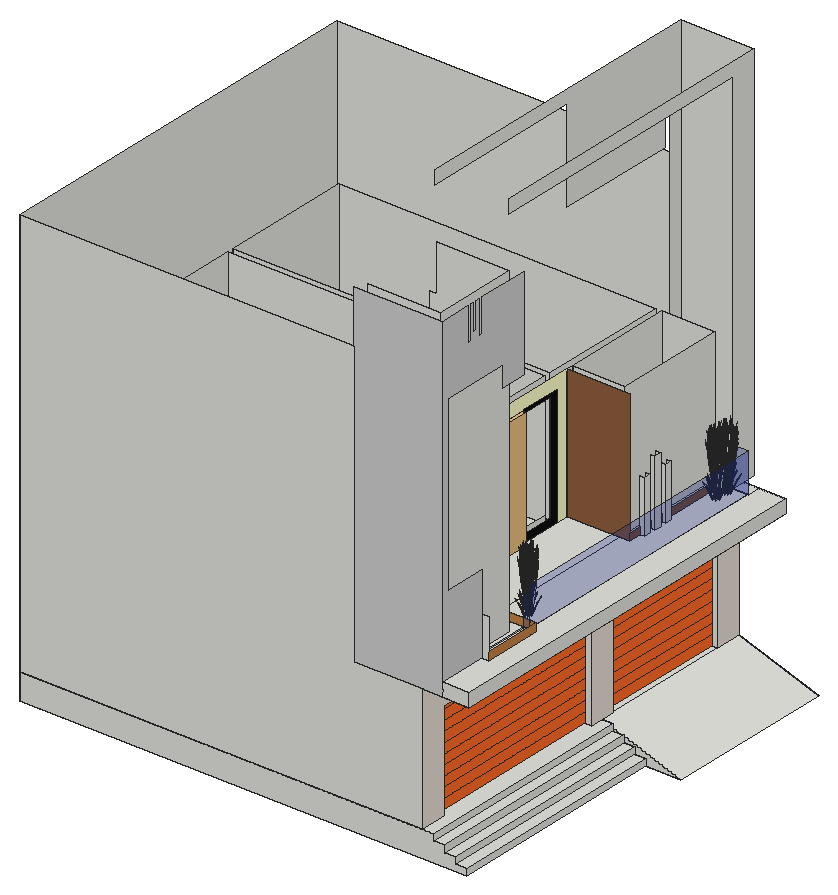
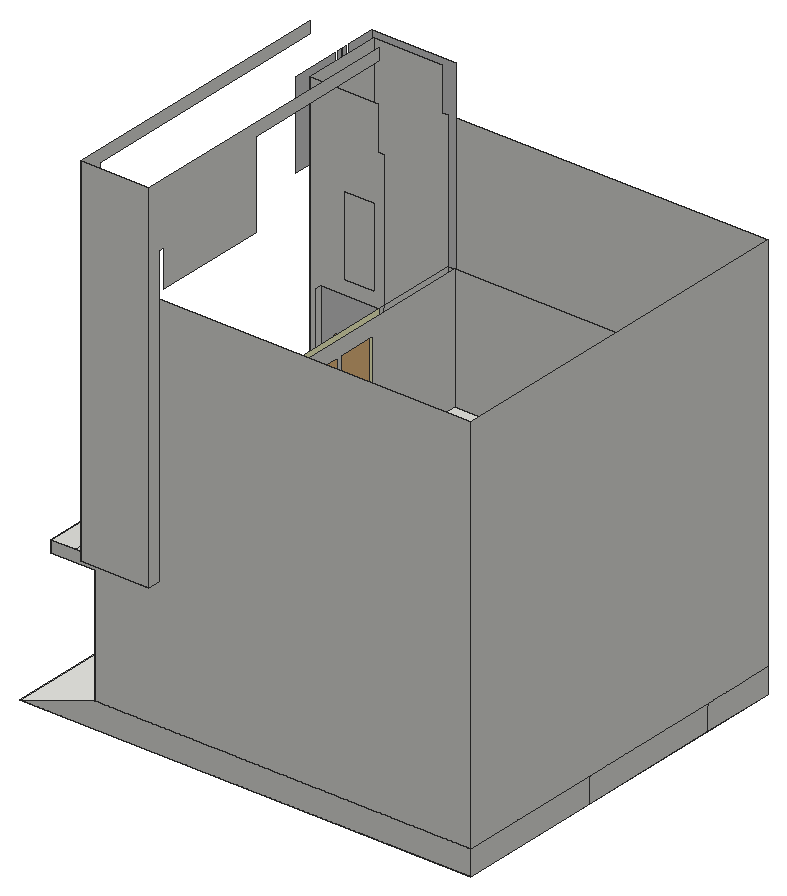
# SketchUp Ruby script. Lengths in inches.
U = 1.inch
M = Sketchup.active_model
def pt(a) = Geom::Point3d.new(a.map { |v| v * U })
def face(e, loops, mat)
  f = e.add_face(loops[0].map { |a| pt(a) })
  loops[1..].each { |l| e.add_face(l.map { |a| pt(a) }).erase! }
  f.material = f.back_material = mat if mat
  f
end
# faces: each face lists its corners as indices into pts; further lists are holes
def faces(e, pts, list, mat = nil) = list.each { |f| face(e, (f[0].is_a?(Array) ? f : [f]).map { |l| l.map { |i| pts[i] } }, mat) }
# xy, xz, yz: faces in a plane at the given z, y or x. An outline is a flat list of corners, or four numbers for a rectangle; further outlines are holes
def ring(l) = l.size == 4 ? [[l[0], l[1]], [l[2], l[1]], [l[2], l[3]], [l[0], l[3]]] : l.each_slice(2).to_a
def flat(e, list, mat, &to3) = list.each { |f| face(e, (f[0].is_a?(Array) ? f : [f]).map { |l| ring(l).map { |u, v| to3.(u, v) } }, mat) }
def xy(e, z, list, mat = nil) = flat(e, list, mat) { |x, y| [x, y, z] }
def xz(e, y, list, mat = nil) = flat(e, list, mat) { |x, z| [x, y, z] }
def yz(e, x, list, mat = nil) = flat(e, list, mat) { |y, z| [x, y, z] }
def lines(e, pts, list) = list.each { |a, b| e.add_line(pt(pts[a]), pt(pts[b])) }
# prism: a flat outline (further loops are holes) pulled along v
def prism(e, loops, v, mat = nil)
  f = face(e, loops, mat); d = Geom::Vector3d.new(v.map { |x| x * U })
  f.pushpull(f.normal.samedirection?(d) ? d.length : -d.length)
end
def box(e, o, s, mat = nil) = prism(e, [[o, [o[0] + s[0], o[1], o[2]], [o[0] + s[0], o[1] + s[1], o[2]], [o[0], o[1] + s[1], o[2]]]], [0, 0, s[2]], mat)
def at(x, y, z, deg = 0) = Geom::Transformation.translation(pt([x, y, z])) * Geom::Transformation.rotation(ORIGIN, Z_AXIS, deg.degrees)
def axes(o, x, y, z) = Geom::Transformation.new([*x, 0, *y, 0, *z, 0, *pt(o).to_a, 1])
def part(name) = M.definitions.add(name)
# library, detail: a bought-in or finely detailed component or shape, given as its bounding box
def library(name, o, s) = part(name).tap { |d| box(d.entities, o, s) }
def detail(e, o, s) = box(e.add_group.entities, o, s)
def put(e, d, t, mat = nil) = e.add_instance(d, t).tap { |i| i.material = mat if mat }
def group(e, t, mat = nil) = e.add_group.tap { |g| g.transformation = t; g.material = mat if mat }.entities
root = M.entities
M.materials.add("C05_Golden_Blaze").color = [255, 107, 39]
M.materials.add("E01_Mint_Frost").color = [255, 255, 204]
M.materials.add("Glass_Basic_01").color = [23, 48, 186]
M.materials["Glass_Basic_01"].alpha = 0.25
M.materials.add("LightPink_Translucent").color = [144, 107, 117]
M.materials["LightPink_Translucent"].alpha = 0.75
M.materials.add("Marble_01_1K").color = [230, 221, 211]
M.materials.add("ThomThom - ShoesRubber1").color = [15, 15, 15]
M.materials.add("Wood_Floor_01_1K").color = [196, 130, 70]
M.materials.add("Wood_Veneer_15_1K").color = [142, 95, 62]
M.materials.add("[Cladding_Siding_White]1").color = [207, 207, 207]
c1 = library("mesh-166",[-1553.69,-2604.3125,-42.18],[1702.88,1401.6,88.28])
c2 = part("Group17\#1")
put(c2.entities,c1,at(294.66,859.51,3.5))
c3 = library("porta+4",[0.2,-5.42,1.33],[46.55,4.72,83.21])
c4 = part("blade")
p = [[2.15,0.21,22],[0,0.17,0],[0.09,0.45,0],[2.18,0.31,22],[2.29,0.31,22],[0.38,0.45,0],
  [2.48,0.24,33],[2.49,0.24,33],[2.48,0.22,33]]
faces(c4.entities,p,[[0,1,2,3],[4,5,2,3],[6,3,4,7],[8,0,3,6]])
c5 = part("seeds")
p = [[0.3,-0.1,1.38],[-0.01,-0.03,1.59],[-0.01,-0.03,0.03],[0.14,-0.07,-0.07],[0.29,-0.03,3],[0.15,0.01,3.11]]
faces(c5.entities,p,[[0,1,2,3],[1,0,4,5]],"LightPink_Translucent")
c6 = part("blade with seeds")
put(c6.entities,c4,at(0,0,0))
put(c6.entities,c5,axes([2.4,0.25,30.99],[1.5799,-0.05474,1.17369],[-0.12525,1.92788,0.29478],[-0.07173,-0.02425,1.56792]))
xy(root,24,[[0,0,0,360,366,360,366,336,360,336,360,216,366,216,366,192,360,192,360,24,366,24,366,0]])
xy(root,114,[[360,24,366,192],[360,216,366,336]])
xy(root,138,[[366,0,408,360]])
xy(root,150,[[384,0,408,0,408,360,384,360,384,99,390,99,390,45,384,45],[9,9,297,225],[303,9,375,87],[303,93,351,243],[351,93,360,93,360,99,384,99,384,348,360,348,360,285,364,285,364,279,360,279,360,273,364,273,364,267,360,267,360,261,364,261,364,255,360,255,360,243,351,243],
  [9,231,297,351],[303,249,351,351],[370,348,384,360],[303,360,370,372]])
xz(root,0,[[0,24,366,24,366,138,303,138,303,396,0,396],[384,138,408,150]])
xz(root,0,[[303,138,384,444]],"[Cladding_Siding_White]1")
xz(root,9,[[9,150,297,270],[297,150,303,270],[303,150,303,402,309,402,309,444,375,444,375,150]])
xz(root,24,[[360,24,366,114]])
xz(root,45,[[384,150,390,186]])
xz(root,87,[[[303,150,375,150,375,444,309,444,309,402,303,402],[312,279,342,357],[312,153,342,231]]])
xz(root,93,[[303,150,303,270,360,270,360,150,345,150,345,234,309,234,309,150],[[309,150,345,234],[312,153,342,231]]],"[Cladding_Siding_White]1")
xz(root,99,[[360,150,384,157],[384,150,390,157]],"Wood_Floor_01_1K")
xz(root,192,[[360,24,366,114]])
xz(root,216,[[360,24,366,114]])
xz(root,225,[[9,150,297,270]])
xz(root,231,[[9,150,297,270]])
xz(root,243,[[303,150,360,270]],"Wood_Veneer_15_1K")
xz(root,249,[[303,150,351,270]])
xz(root,255,[[360,150,364,198]])
xz(root,261,[[360,150,364,198]])
xz(root,267,[[360,150,364,210]])
xz(root,273,[[360,150,364,210]])
xz(root,279,[[360,150,364,198]])
xz(root,285,[[360,150,364,198]])
xz(root,336,[[360,24,366,114]])
xz(root,348,[[360,150,370,186]])
xz(root,348,[[370,150,384,186]],"Glass_Basic_01")
xz(root,351,[[9,150,297,270],[303,150,351,270]])
xz(root,360,[[0,24,0,396,303,396,303,150,408,150,408,138,366,138,366,24]])
xz(root,372,[[303,150,370,498]])
yz(root,0,[[0,24,360,396]])
yz(root,9,[[9,150,225,270],[231,150,351,270]])
yz(root,297,[[[9,150,9,270,225,270,225,255.54,192,255.54,192,156.54,225,156.54,225,150],[108,156.54,147,255.54],[151,156.54,188,255.54]],[231,150,351,270]])
yz(root,303,[[9,150,87,270],[87,150,93,270],[360,150,360,438,354,438,354,402,243,402,243,486,93,486,93,498,372,498,372,150],[243,150,249,270],[249,150,351,270]])
yz(root,303,[[93,150,192,150,192,186.54,188,186.54,188,156.54,151,156.54,151,186.54,147,186.54,147,156.54,108,156.54,108,186.54,105,186.54,105,258.54,231,258.54,231,150,243,150,243,270,93,270]],"E01_Mint_Frost")
yz(root,303,[[192,150,231,150,231,258.51,192,258.51,192,255.54,225,255.54,225,156.54,192,156.54]],"ThomThom - ShoesRubber1")
yz(root,351,[[249,150,351,270]])
yz(root,360,[[93,150,99,270]])
yz(root,360,[[24,24,192,33],[216,24,336,33],[24,33,192,42],[216,33,336,42],[24,42,192,51],
  [216,42,336,51],[24,51,192,60],[216,51,336,60],[24,60,192,69],[216,60,336,69],
  [24,69,192,78],[216,69,336,78],[24,78,192,87],[216,78,336,87],[24,87,192,96],
  [216,87,336,96],[24,96,192,105],[216,96,336,105],[24,105,192,114],[216,105,336,114]],"C05_Golden_Blaze")
yz(root,360,[[243,150,255,156],[261,150,267,156],[273,150,279,156],[285,150,348,156]],"Wood_Veneer_15_1K")
yz(root,364,[[255,150,261,198],[267,150,273,210],[279,150,285,198]])
yz(root,366,[[0,24,24,24,24,114,192,114,192,24,216,24,216,114,336,114,336,24,360,24,360,138,0,138]],"Marble_01_1K")
yz(root,370,[[348,150,372,150,372,498,93,498,93,486,348,486]])
yz(root,375,[[9,150,87,444]])
yz(root,384,[[93,150,99,180],[99,150,348,186]],"Glass_Basic_01")
yz(root,384,[[0,150,45,150,45,222,6,222,6,378,69,378,69,360,93,360,93,444,45.12,444,45.12,414,41.79,414,41.79,444,38.45,444,38.45,420,35.12,420,35.12,444,31.79,444,31.79,414,28.45,414,28.45,444,0,444]],"[Cladding_Siding_White]1")
yz(root,390,[[45,150,99,157]],"Wood_Floor_01_1K")
yz(root,408,[[0,138,360,150]])
p = [[384,93,150],[390,93,150],[303,231,150],[303.15,190.71,150],[303.15,190.71,258.51],[360,242.96,150],
  [360,243,150],[360,255,150],[360,261,150],[360,267,150],[360,273,150],[360,279,150],
  [360,285,150]]
lines(root,p,[[0,1],[2,3],[3,4],[5,6],[7,8],[9,10],[11,12]])
g1 = group(root,at(0,0,0))
xy(g1,0,[[0,0,0,360,366,360,366,204,406,204,406,0],[366,204,438,360]])
xy(g1,6,[[396,0,406,204]])
xy(g1,12,[[386,0,396,204]])
xy(g1,18,[[376,0,386,204]])
xy(g1,24,[[0,0,376,0,376,204,366,204,366,360,0,360]])
xz(g1,0,[[0,0,406,0,406,6,396,6,396,12,386,12,386,18,376,18,376,24,0,24]])
xz(g1,204,[[366,0,406,6],[406,0,438,0,386,17.33,386,12,396,12,396,6,406,6],[366,6,396,12],[366,12,366,18,384,18,386,17.33,386,12],[386,17.33,384,18,386,18],
  [366,18,366,24,376,20.67,376,18],[376,18,376,20.67,384,18],[376,20.67,366,24,376,24]])
xz(g1,360,[[0,0,0,24,366,24,438,0]])
yz(g1,0,[[0,0,72,24],[72,0,216,24],[216,0,360,24]])
yz(g1,376,[[0,18,204,24]])
yz(g1,386,[[0,12,204,18]])
yz(g1,396,[[0,6,204,12]])
yz(g1,406,[[0,0,204,6]])
p = [[376,204,20.67],[384,204,18],[386,204,17.33],[438,204,0],[438,360,0],[366,360,24],
  [366,204,24]]
faces(g1,p,[[0,1,2,3,4,5,6]])
put(root,c2,axes([304.95,127.5625,285.12],[0,-0.05083,0],[0,0,0.07744],[-0.03937,0,0]))
put(root,c3,axes([310,97.01,148.65],[0.74,0,0],[0,0.74,0],[0,0,1.01007]))
put(root,c6,axes([370.13,327.31,151.97],[-0.2011,-0.61905,-0.65645],[0.5793,-0.22295,-0.17229],[-0.02223,-0.20963,1.449]))
put(root,c6,axes([371.39,112.01,151.97],[-0.2011,-0.61905,-0.65645],[0.5793,-0.22295,-0.17229],[-0.02223,-0.20963,1.449]))
put(root,c6,axes([371.39,338.93,151.97],[-0.2011,-0.61905,-0.65645],[0.5793,-0.22295,-0.17229],[-0.02223,-0.20963,1.449]))
put(root,c6,axes([371.97,328.36,151.97],[0.17956,0.55272,-0.65059],[-0.51723,0.19906,-0.17075],[0.01985,0.18717,1.43607]))
put(root,c6,axes([373.23,113.07,151.97],[0.17956,0.55272,-0.65059],[-0.51723,0.19906,-0.17075],[0.01985,0.18717,1.43607]))
put(root,c6,axes([373.23,339.99,151.97],[0.17956,0.55272,-0.65059],[-0.51723,0.19906,-0.17075],[0.01985,0.18717,1.43607]))
put(root,c6,axes([371.92,327.2,151.9375],[0.50939,0.09897,-0.58612],[-0.10749,0.61051,-0.15383],[0.15202,0.07398,1.29375]))
put(root,c6,axes([370.21,328.46,151.9375],[-0.50939,-0.09897,-0.58612],[0.10749,-0.61051,-0.15383],[-0.15202,-0.07398,1.29375]))
put(root,c6,axes([371.01,326.67,151.9375],[0.32983,-0.45375,-0.58612],[0.40974,0.41145,-0.15383],[0.13217,-0.11319,1.29375]))
put(root,c6,axes([371.12,328.99,151.9375],[-0.32983,0.45375,-0.58612],[-0.40974,-0.41145,-0.15383],[-0.13217,0.11319,1.29375]))
put(root,c6,axes([373.18,111.91,151.9375],[0.50939,0.09897,-0.58612],[-0.10749,0.61051,-0.15383],[0.15202,0.07398,1.29375]))
put(root,c6,axes([371.47,113.17,151.9375],[-0.50939,-0.09897,-0.58612],[0.10749,-0.61051,-0.15383],[-0.15202,-0.07398,1.29375]))
put(root,c6,axes([372.27,111.38,151.9375],[0.32983,-0.45375,-0.58612],[0.40974,0.41145,-0.15383],[0.13217,-0.11319,1.29375]))
put(root,c6,axes([372.375,113.7,151.9375],[-0.32983,0.45375,-0.58612],[-0.40974,-0.41145,-0.15383],[-0.13217,0.11319,1.29375]))
put(root,c6,axes([373.18,338.83,151.9375],[0.50939,0.09897,-0.58612],[-0.10749,0.61051,-0.15383],[0.15202,0.07398,1.29375]))
put(root,c6,axes([371.47,340.09,151.9375],[-0.50939,-0.09897,-0.58612],[0.10749,-0.61051,-0.15383],[-0.15202,-0.07398,1.29375]))
put(root,c6,axes([372.27,338.3,151.9375],[0.32983,-0.45375,-0.58612],[0.40974,0.41145,-0.15383],[0.13217,-0.11319,1.29375]))
put(root,c6,axes([372.375,340.62,151.9375],[-0.32983,0.45375,-0.58612],[-0.40974,-0.41145,-0.15383],[-0.13217,0.11319,1.29375]))
put(root,c6,axes([372.59,326.04,151.9],[0.4583,0.30184,-0.46672],[-0.27394,0.54125,0],[0.10438,0.06875,1.48054]))
put(root,c6,axes([371.66,330.23,151.9],[-0.4583,0.30184,-0.46672],[-0.27394,-0.54125,0],[-0.10438,0.06875,1.48054]))
put(root,c6,axes([368.95,327.22,151.9],[0,-0.60368,-0.46672],[0.54787,0,0],[0,-0.13749,1.48054]))
put(root,c6,axes([369.54,329.62,151.9],[-0.4583,-0.30184,-0.46672],[0.27394,-0.54125,0],[-0.10438,-0.06875,1.48054]))
put(root,c6,axes([370.47,325.43,151.9],[0.4583,-0.30184,-0.46672],[0.27394,0.54125,0],[0.10438,-0.06875,1.48054]))
put(root,c6,axes([373.18,328.4375,151.9],[0,0.60368,-0.46672],[-0.54787,0,0],[0,0.13749,1.48054]))
put(root,c6,axes([373.85,110.75,151.9],[0.4583,0.30184,-0.46672],[-0.27394,0.54125,0],[0.10438,0.06875,1.48054]))
put(root,c6,axes([372.92,114.94,151.9],[-0.4583,0.30184,-0.46672],[-0.27394,-0.54125,0],[-0.10438,0.06875,1.48054]))
put(root,c6,axes([370.21,111.93,151.9],[0,-0.60368,-0.46672],[0.54787,0,0],[0,-0.13749,1.48054]))
put(root,c6,axes([370.8,114.32,151.9],[-0.4583,-0.30184,-0.46672],[0.27394,-0.54125,0],[-0.10438,-0.06875,1.48054]))
put(root,c6,axes([371.73,110.14,151.9],[0.4583,-0.30184,-0.46672],[0.27394,0.54125,0],[0.10438,-0.06875,1.48054]))
put(root,c6,axes([374.44,113.15,151.9],[0,0.60368,-0.46672],[-0.54787,0,0],[0,0.13749,1.48054]))
put(root,c6,axes([373.85,337.67,151.9],[0.4583,0.30184,-0.46672],[-0.27394,0.54125,0],[0.10438,0.06875,1.48054]))
put(root,c6,axes([372.92,341.85,151.9],[-0.4583,0.30184,-0.46672],[-0.27394,-0.54125,0],[-0.10438,0.06875,1.48054]))
put(root,c6,axes([370.21,338.85,151.9],[0,-0.60368,-0.46672],[0.54787,0,0],[0,-0.13749,1.48054]))
put(root,c6,axes([370.8,341.24,151.9],[-0.4583,-0.30184,-0.46672],[0.27394,-0.54125,0],[-0.10438,-0.06875,1.48054]))
put(root,c6,axes([371.73,337.06,151.9],[0.4583,-0.30184,-0.46672],[0.27394,0.54125,0],[0.10438,-0.06875,1.48054]))
put(root,c6,axes([374.44,340.07,151.9],[0,0.60368,-0.46672],[-0.54787,0,0],[0,0.13749,1.48054]))
put(root,c6,axes([370.4375,327.47,152.08],[0.23759,-0.54397,-0.42055],[0.49367,0.26179,0.2024],[0,-0.12539,1.35025]))
put(root,c6,axes([370.47,328.27,152.08],[-0.29417,-0.5067,-0.42055],[0.44558,-0.35681,0.2024],[-0.0952,-0.0627,1.35025]))
put(root,c6,axes([371.65,327.39,152.08],[0.29417,0.5067,-0.42055],[-0.44558,0.35681,0.2024],[0.0952,0.0627,1.35025]))
put(root,c6,axes([371.69,328.19,152.08],[-0.23759,0.54397,-0.42055],[-0.49367,-0.26179,0.2024],[0,0.12539,1.35025]))
put(root,c6,axes([371.1,328.63,152.08],[-0.53176,0.03727,-0.42055],[-0.04809,-0.6186,0.2024],[-0.0952,0.0627,1.35025]))
put(root,c6,axes([371.7,112.17,152.08],[0.23759,-0.54397,-0.42055],[0.49367,0.26179,0.2024],[0,-0.12539,1.35025]))
put(root,c6,axes([371.73,112.98,152.08],[-0.29417,-0.5067,-0.42055],[0.44558,-0.35681,0.2024],[-0.0952,-0.0627,1.35025]))
put(root,c6,axes([372.91,112.1,152.08],[0.29417,0.5067,-0.42055],[-0.44558,0.35681,0.2024],[0.0952,0.0627,1.35025]))
put(root,c6,axes([372.95,112.9,152.08],[-0.23759,0.54397,-0.42055],[-0.49367,-0.26179,0.2024],[0,0.12539,1.35025]))
put(root,c6,axes([372.36,113.34,152.08],[-0.53176,0.03727,-0.42055],[-0.04809,-0.6186,0.2024],[-0.0952,0.0627,1.35025]))
put(root,c6,axes([371.7,339.09,152.08],[0.23759,-0.54397,-0.42055],[0.49367,0.26179,0.2024],[0,-0.12539,1.35025]))
put(root,c6,axes([371.73,339.89,152.08],[-0.29417,-0.5067,-0.42055],[0.44558,-0.35681,0.2024],[-0.0952,-0.0627,1.35025]))
put(root,c6,axes([372.91,339.02,152.08],[0.29417,0.5067,-0.42055],[-0.44558,0.35681,0.2024],[0.0952,0.0627,1.35025]))
put(root,c6,axes([372.95,339.82,152.08],[-0.23759,0.54397,-0.42055],[-0.49367,-0.26179,0.2024],[0,0.12539,1.35025]))
put(root,c6,axes([372.36,340.26,152.08],[-0.53176,0.03727,-0.42055],[-0.04809,-0.6186,0.2024],[-0.0952,0.0627,1.35025]))
put(root,c6,axes([370.58,325.67,151.91],[0.45686,0.14937,-0.29119],[-0.11503,0.52602,0.29119],[0.0921,-0.06066,1.30635]))
put(root,c6,axes([372.95,328.43,151.91],[-0.34183,0.37665,-0.29119],[-0.34183,-0.37665,0.29119],[0,0.12132,1.30635]))
put(root,c6,axes([369.67,329.39,151.91],[-0.11503,-0.52602,-0.29119],[0.45686,-0.14937,0.29119],[-0.0921,-0.06066,1.30635]))
put(root,c6,axes([371.55,329.99,151.91],[-0.45686,-0.14937,-0.29119],[0.11503,-0.52602,0.29119],[-0.0921,0.06066,1.30635]))
put(root,c6,axes([372.46,326.27,151.91],[0.11503,0.52602,-0.29119],[-0.45686,0.14937,0.29119],[0.0921,0.06066,1.30635]))
put(root,c6,axes([369.18,327.23,151.91],[0.34183,-0.37665,-0.29119],[0.34183,0.37665,0.29119],[0,-0.12132,1.30635]))
put(root,c6,axes([371.84,110.38,151.91],[0.45686,0.14937,-0.29119],[-0.11503,0.52602,0.29119],[0.0921,-0.06066,1.30635]))
put(root,c6,axes([374.21,113.13,151.91],[-0.34183,0.37665,-0.29119],[-0.34183,-0.37665,0.29119],[0,0.12132,1.30635]))
put(root,c6,axes([370.93,114.1,151.91],[-0.11503,-0.52602,-0.29119],[0.45686,-0.14937,0.29119],[-0.0921,-0.06066,1.30635]))
put(root,c6,axes([372.8125,114.7,151.91],[-0.45686,-0.14937,-0.29119],[0.11503,-0.52602,0.29119],[-0.0921,0.06066,1.30635]))
put(root,c6,axes([373.72,110.98,151.91],[0.11503,0.52602,-0.29119],[-0.45686,0.14937,0.29119],[0.0921,0.06066,1.30635]))
put(root,c6,axes([370.44,111.94,151.91],[0.34183,-0.37665,-0.29119],[0.34183,0.37665,0.29119],[0,-0.12132,1.30635]))
put(root,c6,axes([371.84,337.3,151.91],[0.45686,0.14937,-0.29119],[-0.11503,0.52602,0.29119],[0.0921,-0.06066,1.30635]))
put(root,c6,axes([374.21,340.05,151.91],[-0.34183,0.37665,-0.29119],[-0.34183,-0.37665,0.29119],[0,0.12132,1.30635]))
put(root,c6,axes([370.93,341.02,151.91],[-0.11503,-0.52602,-0.29119],[0.45686,-0.14937,0.29119],[-0.0921,-0.06066,1.30635]))
put(root,c6,axes([372.8125,341.62,151.91],[-0.45686,-0.14937,-0.29119],[0.11503,-0.52602,0.29119],[-0.0921,0.06066,1.30635]))
put(root,c6,axes([373.72,337.9,151.91],[0.11503,0.52602,-0.29119],[-0.45686,0.14937,0.29119],[0.0921,0.06066,1.30635]))
put(root,c6,axes([370.44,338.86,151.91],[0.34183,-0.37665,-0.29119],[0.34183,0.37665,0.29119],[0,-0.12132,1.30635]))
put(root,c6,axes([372.5625,330.34,151.4],[0.03568,-0.08715,1.65762],[0.44916,-0.25668,-0.25323],[0.13617,0.13285,0.28235]))
put(root,c6,axes([368.57,327.6,151.4],[0.01242,0.09514,1.65762],[-0.25036,0.49684,-0.25323],[-0.17783,-0.02504,0.28235]))
put(root,c6,axes([370.81,324.37,151.4],[-0.08214,0.02175,1.65762],[-0.45422,-0.24483,-0.25323],[0.00762,-0.20421,0.28235]))
put(root,c6,axes([370.47,330.32,151.4],[0.07925,-0.03285,1.65762],[0.47671,0.18081,-0.25323],[0.01394,0.20378,0.28235]))
put(root,c6,axes([373.86,327.69,151.4],[-0.02559,-0.09165,1.65762],[0.1775,-0.53611,-0.25323],[0.17905,-0.00771,0.28235]))
put(root,c6,axes([369.34,325.12,151.4],[-0.04743,0.07953,1.65762],[-0.47936,0.17146,-0.25323],[-0.1158,-0.15598,0.28235]))
put(root,c6,axes([368.4375,330.26,151.4],[0.06569,0.06031,1.65762],[0.11138,0.55882,-0.25323],[-0.14558,0.11917,0.28235]))
put(root,c6,axes([372.82,325.41,151.4],[-0.07329,-0.04756,1.65762],[-0.18827,-0.53132,-0.25323],[0.127,-0.14418,0.28235]))
put(root,c6,axes([373.82,115.05,151.4],[0.03568,-0.08715,1.65762],[0.44916,-0.25668,-0.25323],[0.13617,0.13285,0.28235]))
put(root,c6,axes([369.83,112.31,151.4],[0.01242,0.09514,1.65762],[-0.25036,0.49684,-0.25323],[-0.17783,-0.02504,0.28235]))
put(root,c6,axes([372.07,109.08,151.4],[-0.08214,0.02175,1.65762],[-0.45422,-0.24483,-0.25323],[0.00762,-0.20421,0.28235]))
put(root,c6,axes([371.73,115.03,151.4],[0.07925,-0.03285,1.65762],[0.47671,0.18081,-0.25323],[0.01394,0.20378,0.28235]))
put(root,c6,axes([375.12,112.4,151.4],[-0.02559,-0.09165,1.65762],[0.1775,-0.53611,-0.25323],[0.17905,-0.00771,0.28235]))
put(root,c6,axes([370.6,109.83,151.4],[-0.04743,0.07953,1.65762],[-0.47936,0.17146,-0.25323],[-0.1158,-0.15598,0.28235]))
put(root,c6,axes([369.7,114.97,151.4],[0.06569,0.06031,1.65762],[0.11138,0.55882,-0.25323],[-0.14558,0.11917,0.28235]))
put(root,c6,axes([374.08,110.12,151.4],[-0.07329,-0.04756,1.65762],[-0.18827,-0.53132,-0.25323],[0.127,-0.14418,0.28235]))
put(root,c6,axes([373.82,341.96,151.4],[0.03568,-0.08715,1.65762],[0.44916,-0.25668,-0.25323],[0.13617,0.13285,0.28235]))
put(root,c6,axes([369.83,339.23,151.4],[0.01242,0.09514,1.65762],[-0.25036,0.49684,-0.25323],[-0.17783,-0.02504,0.28235]))
put(root,c6,axes([372.07,336,151.4],[-0.08214,0.02175,1.65762],[-0.45422,-0.24483,-0.25323],[0.00762,-0.20421,0.28235]))
put(root,c6,axes([371.73,341.95,151.4],[0.07925,-0.03285,1.65762],[0.47671,0.18081,-0.25323],[0.01394,0.20378,0.28235]))
put(root,c6,axes([375.12,339.32,151.4],[-0.02559,-0.09165,1.65762],[0.1775,-0.53611,-0.25323],[0.17905,-0.00771,0.28235]))
put(root,c6,axes([370.6,336.75,151.4],[-0.04743,0.07953,1.65762],[-0.47936,0.17146,-0.25323],[-0.1158,-0.15598,0.28235]))
put(root,c6,axes([369.7,341.89,151.4],[0.06569,0.06031,1.65762],[0.11138,0.55882,-0.25323],[-0.14558,0.11917,0.28235]))
put(root,c6,axes([374.08,337.04,151.4],[-0.07329,-0.04756,1.65762],[-0.18827,-0.53132,-0.25323],[0.127,-0.14418,0.28235]))
put(root,c6,axes([370.09,326.75,151.5],[-0.482,0.24169,1.21193],[-0.15342,-0.69348,0.47091],[0.29598,0.01154,1.37843]))
put(root,c6,axes([371.35,111.46,151.5],[-0.482,0.24169,1.21193],[-0.15342,-0.69348,0.47091],[0.29598,0.01154,1.37843]))
put(root,c6,axes([371.35,338.38,151.5],[-0.482,0.24169,1.21193],[-0.15342,-0.69348,0.47091],[0.29598,0.01154,1.37843]))
put(root,c6,axes([371.47,328.46,152.51],[0.05706,0.68884,-0.2735],[-0.59432,0.04165,-0.47002],[-0.10465,0.09176,1.50125]))
put(root,c6,axes([371.75,327.74,152.51],[0.55148,0.28805,-0.2735],[-0.26554,0.60796,-0.47002],[0.01733,0.14927,1.50125]))
put(root,c6,axes([370.38,327.92,152.51],[-0.55148,-0.28805,-0.2735],[0.26554,-0.60796,-0.47002],[-0.01733,-0.14927,1.50125]))
put(root,c6,axes([370.65,327.2,152.51],[-0.05706,-0.68884,-0.2735],[0.59432,-0.04165,-0.47002],[0.10465,-0.09176,1.50125]))
put(root,c6,axes([371.34,327.11,152.51],[0.49442,-0.40079,-0.2735],[0.32878,0.56631,-0.47002],[0.12199,0.05751,1.50125]))
put(root,c6,axes([370.79,328.55,152.51],[-0.49442,0.40079,-0.2735],[-0.32878,-0.56631,-0.47002],[-0.12199,-0.05751,1.50125]))
put(root,c6,axes([372.73,113.17,152.51],[0.05706,0.68884,-0.2735],[-0.59432,0.04165,-0.47002],[-0.10465,0.09176,1.50125]))
put(root,c6,axes([373.01,112.45,152.51],[0.55148,0.28805,-0.2735],[-0.26554,0.60796,-0.47002],[0.01733,0.14927,1.50125]))
put(root,c6,axes([371.64,112.625,152.51],[-0.55148,-0.28805,-0.2735],[0.26554,-0.60796,-0.47002],[-0.01733,-0.14927,1.50125]))
put(root,c6,axes([371.91,111.9,152.51],[-0.05706,-0.68884,-0.2735],[0.59432,-0.04165,-0.47002],[0.10465,-0.09176,1.50125]))
put(root,c6,axes([372.6,111.82,152.51],[0.49442,-0.40079,-0.2735],[0.32878,0.56631,-0.47002],[0.12199,0.05751,1.50125]))
put(root,c6,axes([372.05,113.26,152.51],[-0.49442,0.40079,-0.2735],[-0.32878,-0.56631,-0.47002],[-0.12199,-0.05751,1.50125]))
put(root,c6,axes([372.73,340.09,152.51],[0.05706,0.68884,-0.2735],[-0.59432,0.04165,-0.47002],[-0.10465,0.09176,1.50125]))
put(root,c6,axes([373.01,339.37,152.51],[0.55148,0.28805,-0.2735],[-0.26554,0.60796,-0.47002],[0.01733,0.14927,1.50125]))
put(root,c6,axes([371.64,339.55,152.51],[-0.55148,-0.28805,-0.2735],[0.26554,-0.60796,-0.47002],[-0.01733,-0.14927,1.50125]))
put(root,c6,axes([371.91,338.82,152.51],[-0.05706,-0.68884,-0.2735],[0.59432,-0.04165,-0.47002],[0.10465,-0.09176,1.50125]))
put(root,c6,axes([372.6,338.74,152.51],[0.49442,-0.40079,-0.2735],[0.32878,0.56631,-0.47002],[0.12199,0.05751,1.50125]))
put(root,c6,axes([372.05,340.18,152.51],[-0.49442,0.40079,-0.2735],[-0.32878,-0.56631,-0.47002],[-0.12199,-0.05751,1.50125]))
put(root,c6,axes([371.64,329.15,152.05],[0.51411,-0.20483,-0.18046],[0.18065,0.59003,0.00007],[0.05675,-0.02264,1.63463]))
put(root,c6,axes([372.9,113.85,152.05],[0.51411,-0.20483,-0.18046],[0.18065,0.59003,0.00007],[0.05675,-0.02264,1.63463]))
put(root,c6,axes([372.9,340.77,152.05],[0.51411,-0.20483,-0.18046],[0.18065,0.59003,0.00007],[0.05675,-0.02264,1.63463]))
put(root,c6,axes([371.34,328.73,152.32],[-0.47817,-0.48589,-0.23681],[0.40236,-0.54561,0.51822],[-0.12876,0.05684,1.58123]))
put(root,c6,axes([372.6,113.44,152.32],[-0.47817,-0.48589,-0.23681],[0.40236,-0.54561,0.51822],[-0.12876,0.05684,1.58123]))
put(root,c6,axes([372.6,340.36,152.32],[-0.47817,-0.48589,-0.23681],[0.40236,-0.54561,0.51822],[-0.12876,0.05684,1.58123]))
put(root,c6,axes([370.52,328.56,152.29],[0.12979,-0.71533,-0.22023],[0.6154,0.12469,0.48194],[-0.10753,-0.09879,1.47054]))
put(root,c6,axes([371.78,113.27,152.29],[0.12979,-0.71533,-0.22023],[0.6154,0.12469,0.48194],[-0.10753,-0.09879,1.47054]))
put(root,c6,axes([371.78,340.19,152.29],[0.12979,-0.71533,-0.22023],[0.6154,0.12469,0.48194],[-0.10753,-0.09879,1.47054]))
put(root,c6,axes([370.72,324.8,152],[-0.3384,0.34633,-0.03659],[-0.31006,-0.3793,-0.1659],[-0.02183,-0.10747,0.54722]))
put(root,c6,axes([369.04,325.43,152],[-0.14126,0.49294,-0.03659],[-0.43477,-0.15163,-0.1659],[-0.06601,-0.08063,0.54722]))
put(root,c6,axes([371.99,109.51,152],[-0.3384,0.34633,-0.03659],[-0.31006,-0.3793,-0.1659],[-0.02183,-0.10747,0.54722]))
put(root,c6,axes([370.3,110.14,152],[-0.14126,0.49294,-0.03659],[-0.43477,-0.15163,-0.1659],[-0.06601,-0.08063,0.54722]))
put(root,c6,axes([371.99,336.42,152],[-0.3384,0.34633,-0.03659],[-0.31006,-0.3793,-0.1659],[-0.02183,-0.10747,0.54722]))
put(root,c6,axes([370.3,337.05,152],[-0.14126,0.49294,-0.03659],[-0.43477,-0.15163,-0.1659],[-0.06601,-0.08063,0.54722]))
put(root,c6,axes([374.09,327.56,152.125],[-0.3036,-0.38602,-0.06098],[0.3325,-0.3537,-0.27651],[0.09421,-0.0249,0.91203]))
put(root,c6,axes([375.35,112.27,152.125],[-0.3036,-0.38602,-0.06098],[0.3325,-0.3537,-0.27651],[0.09421,-0.0249,0.91203]))
put(root,c6,axes([375.35,339.1875,152.125],[-0.3036,-0.38602,-0.06098],[0.3325,-0.3537,-0.27651],[0.09421,-0.0249,0.91203]))
put(root,c6,axes([373.51,328.07,151.86],[-0.3154,0.07245,1.33088],[-0.0502,-0.57666,0.07618],[0.2209,-0.08728,0.75732]))
put(root,c6,axes([374.77,112.78,151.86],[-0.3154,0.07245,1.33088],[-0.0502,-0.57666,0.07618],[0.2209,-0.08728,0.75732]))
put(root,c6,axes([374.77,339.7,151.86],[-0.3154,0.07245,1.33088],[-0.0502,-0.57666,0.07618],[0.2209,-0.08728,0.75732]))
put(root,c6,axes([371.69,330.06,152.0625],[-0.30235,-0.60704,-0.04834],[0.51222,-0.33735,0.48511],[-0.12622,0.0578,1.53813]))
put(root,c6,axes([372.95,114.77,152.0625],[-0.30235,-0.60704,-0.04834],[0.51222,-0.33735,0.48511],[-0.12622,0.0578,1.53813]))
put(root,c6,axes([372.95,341.69,152.0625],[-0.30235,-0.60704,-0.04834],[0.51222,-0.33735,0.48511],[-0.12622,0.0578,1.53813]))
put(root,c6,axes([373.07,328.33,152.07],[-0.61202,-0.00483,-0.04678],[0,-0.67471,0.46946],[-0.01923,0.15359,1.48851]))
put(root,c6,axes([374.33,113.04,152.07],[-0.61202,-0.00483,-0.04678],[0,-0.67471,0.46946],[-0.01923,0.15359,1.48851]))
put(root,c6,axes([374.33,339.96,152.07],[-0.61202,-0.00483,-0.04678],[0,-0.67471,0.46946],[-0.01923,0.15359,1.48851]))
put(root,c6,axes([371.32,329.24,152.15],[0.2129,0.69353,-0.05652],[-0.60833,0.24302,0],[0.00743,0.02422,1.61843]))
put(root,c6,axes([372.58,113.95,152.15],[0.2129,0.69353,-0.05652],[-0.60833,0.24302,0],[0.00743,0.02422,1.61843]))
put(root,c6,axes([372.58,340.87,152.15],[0.2129,0.69353,-0.05652],[-0.60833,0.24302,0],[0.00743,0.02422,1.61843]))
put(root,c6,axes([371.45,328.15,152.16],[-0.45549,-0.5196,-0.05763],[0.45577,-0.51991,0],[-0.01591,-0.01814,1.65037]))
put(root,c6,axes([372.71,112.86,152.16],[-0.45549,-0.5196,-0.05763],[0.45577,-0.51991,0],[-0.01591,-0.01814,1.65037]))
put(root,c6,axes([372.71,339.78,152.16],[-0.45549,-0.5196,-0.05763],[0.45577,-0.51991,0],[-0.01591,-0.01814,1.65037]))
put(root,c6,axes([371.61,327.89,152.15],[0,0.69816,-0.05299],[-0.61233,0,0],[0,0.02194,1.68606]))
put(root,c6,axes([372.87,112.6,152.15],[0,0.69816,-0.05299],[-0.61233,0,0],[0,0.02194,1.68606]))
put(root,c6,axes([372.87,339.51,152.15],[0,0.69816,-0.05299],[-0.61233,0,0],[0,0.02194,1.68606]))
put(root,c6,axes([370.05,325.53,152.23],[-0.30616,-0.60492,0],[0.51222,-0.33735,-0.48511],[0.11666,-0.07683,1.53889]))
put(root,c6,axes([369.82,329.98,152.23],[-0.30616,0.60492,0],[-0.51222,-0.33735,-0.48511],[-0.11666,-0.07683,1.53889]))
put(root,c6,axes([372.08,330.13,152.23],[0.30616,0.60492,0],[-0.51222,0.33735,-0.48511],[-0.11666,0.07683,1.53889]))
put(root,c6,axes([368.81,327.68,152.23],[-0.61233,0,0],[0,-0.67471,-0.48511],[0,-0.15367,1.53889]))
put(root,c6,axes([371.3125,110.23,152.23],[-0.30616,-0.60492,0],[0.51222,-0.33735,-0.48511],[0.11666,-0.07683,1.53889]))
put(root,c6,axes([371.08,114.6875,152.23],[-0.30616,0.60492,0],[-0.51222,-0.33735,-0.48511],[-0.11666,-0.07683,1.53889]))
put(root,c6,axes([373.34,114.84,152.23],[0.30616,0.60492,0],[-0.51222,0.33735,-0.48511],[-0.11666,0.07683,1.53889]))
put(root,c6,axes([370.07,112.39,152.23],[-0.61233,0,0],[0,-0.67471,-0.48511],[0,-0.15367,1.53889]))
put(root,c6,axes([371.3125,337.15,152.23],[-0.30616,-0.60492,0],[0.51222,-0.33735,-0.48511],[0.11666,-0.07683,1.53889]))
put(root,c6,axes([371.08,341.61,152.23],[-0.30616,0.60492,0],[-0.51222,-0.33735,-0.48511],[-0.11666,-0.07683,1.53889]))
put(root,c6,axes([373.34,341.76,152.23],[0.30616,0.60492,0],[-0.51222,0.33735,-0.48511],[-0.11666,0.07683,1.53889]))
put(root,c6,axes([370.07,339.3,152.23],[-0.61233,0,0],[0,-0.67471,-0.48511],[0,-0.15367,1.53889]))
put(root,c6,axes([372.31,325.68,152.23],[0.30616,-0.60492,0],[0.51222,0.33735,-0.48511],[0.11666,0.07683,1.53889]))
put(root,c6,axes([373.32,327.98,152.23],[0.61233,0,0],[0,0.67471,-0.48511],[0,0.15367,1.53889]))
put(root,c6,axes([373.57,110.39,152.23],[0.30616,-0.60492,0],[0.51222,0.33735,-0.48511],[0.11666,0.07683,1.53889]))
put(root,c6,axes([374.58,112.69,152.23],[0.61233,0,0],[0,0.67471,-0.48511],[0,0.15367,1.53889]))
put(root,c6,axes([373.57,337.31,152.23],[0.30616,-0.60492,0],[0.51222,0.33735,-0.48511],[0.11666,0.07683,1.53889]))
put(root,c6,axes([374.58,339.61,152.23],[0.61233,0,0],[0,0.67471,-0.48511],[0,0.15367,1.53889]))
put(root,c6,axes([369.28,327.5,152.19],[-0.45549,0.50754,0.28911],[-0.45577,-0.5022,-0.34302],[-0.01591,-0.14413,1.54992]))
put(root,c6,axes([371.7,329.75,152.19],[0.61306,0.19622,0.28911],[-0.15337,0.70136,-0.34302],[-0.10147,0.08778,1.54992]))
put(root,c6,axes([370.54,112.21,152.19],[-0.45549,0.50754,0.28911],[-0.45577,-0.5022,-0.34302],[-0.01591,-0.14413,1.54992]))
put(root,c6,axes([372.96,114.46,152.19],[0.61306,0.19622,0.28911],[-0.15337,0.70136,-0.34302],[-0.10147,0.08778,1.54992]))
put(root,c6,axes([370.54,339.125,152.19],[-0.45549,0.50754,0.28911],[-0.45577,-0.5022,-0.34302],[-0.01591,-0.14413,1.54992]))
put(root,c6,axes([372.96,341.38,152.19],[0.61306,0.19622,0.28911],[-0.15337,0.70136,-0.34302],[-0.10147,0.08778,1.54992]))
put(root,c6,axes([370.93,329.45,152.0625],[-0.49367,-0.27103,0],[0.23759,-0.56315,0],[0,0,1.52945]))
put(root,c6,axes([372.19,114.16,152.0625],[-0.49367,-0.27103,0],[0.23759,-0.56315,0],[0,0,1.52945]))
put(root,c6,axes([372.19,341.08,152.0625],[-0.49367,-0.27103,0],[0.23759,-0.56315,0],[0,0,1.52945]))
put(root,c6,axes([371.49,329.47,152.07],[0.49367,0.27103,0],[-0.23759,0.56315,0],[0,0,1.64456]))
put(root,c6,axes([372.75,114.17,152.07],[0.49367,0.27103,0],[-0.23759,0.56315,0],[0,0,1.64456]))
put(root,c6,axes([372.75,341.09,152.07],[0.49367,0.27103,0],[-0.23759,0.56315,0],[0,0,1.64456]))
put(root,c6,axes([371.05,329.22,152.07],[-0.15978,-0.52046,0],[0.45625,-0.18226,0],[0,0,1.45109]))
put(root,c6,axes([372.31,113.93,152.07],[-0.15978,-0.52046,0],[0.45625,-0.18226,0],[0,0,1.45109]))
put(root,c6,axes([372.31,340.85,152.07],[-0.15978,-0.52046,0],[0.45625,-0.18226,0],[0,0,1.45109]))
put(root,c6,axes([371.3,327.61,152.07],[0,-0.69851,0],[0.61233,0,0],[0,0,1.68689]))
put(root,c6,axes([372.5625,112.32,152.07],[0,-0.69851,0],[0.61233,0,0],[0,0,1.68689]))
put(root,c6,axes([372.5625,339.24,152.07],[0,-0.69851,0],[0.61233,0,0],[0,0,1.68689]))
put(root,c6,axes([371.72,327.76,152.07],[0.54787,0,0],[0,0.62498,0],[0,0,1.67702]))
put(root,c6,axes([372.98,112.47,152.07],[0.54787,0,0],[0,0.62498,0],[0,0,1.67702]))
put(root,c6,axes([372.98,339.39,152.07],[0.54787,0,0],[0,0.62498,0],[0,0,1.67702]))
put(root,c6,axes([371.7,328.03,152.08],[0.34183,0.38994,0],[-0.34183,0.38994,0],[0,0,1.5911]))
put(root,c6,axes([372.96,112.74,152.08],[0.34183,0.38994,0],[-0.34183,0.38994,0],[0,0,1.5911]))
put(root,c6,axes([372.96,339.66,152.08],[0.34183,0.38994,0],[-0.34183,0.38994,0],[0,0,1.5911]))
put(root,c6,axes([370.59,328.21,152.22],[0.61893,0.12719,0.43009],[-0.12596,0.71835,0.16877],[-0.09045,-0.06936,1.49325]))
put(root,c6,axes([371.01,327.17,152.22],[-0.40602,0.54785,0.43009],[-0.48237,-0.48361,0.16877],[0.09788,-0.05467,1.49325]))
put(root,c6,axes([370.54,327.55,152.22],[0.2129,0.67504,0.43009],[-0.60833,0.23474,0.16877],[0.00743,-0.12404,1.49325]))
put(root,c6,axes([371.85,112.92,152.22],[0.61893,0.12719,0.43009],[-0.12596,0.71835,0.16877],[-0.09045,-0.06936,1.49325]))
put(root,c6,axes([372.27,111.875,152.22],[-0.40602,0.54785,0.43009],[-0.48237,-0.48361,0.16877],[0.09788,-0.05467,1.49325]))
put(root,c6,axes([371.8,112.26,152.22],[0.2129,0.67504,0.43009],[-0.60833,0.23474,0.16877],[0.00743,-0.12404,1.49325]))
put(root,c6,axes([371.85,339.84,152.22],[0.61893,0.12719,0.43009],[-0.12596,0.71835,0.16877],[-0.09045,-0.06936,1.49325]))
put(root,c6,axes([372.27,338.8,152.22],[-0.40602,0.54785,0.43009],[-0.48237,-0.48361,0.16877],[0.09788,-0.05467,1.49325]))
put(root,c6,axes([371.8,339.18,152.22],[0.2129,0.67504,0.43009],[-0.60833,0.23474,0.16877],[0.00743,-0.12404,1.49325]))
put(root,c6,axes([371.54,327.45,152.24],[-0.61893,-0.12719,0.46247],[0.12596,-0.71835,0.18148],[0.09045,0.06936,1.60565]))
put(root,c6,axes([372.8,112.15,152.24],[-0.61893,-0.12719,0.46247],[0.12596,-0.71835,0.18148],[0.09045,0.06936,1.60565]))
put(root,c6,axes([372.8,339.07,152.24],[-0.61893,-0.12719,0.46247],[0.12596,-0.71835,0.18148],[0.09045,0.06936,1.60565]))
put(root,c6,axes([370.73,327.74,152.29],[0.55175,0.29259,0.22621],[-0.26554,0.60796,0.47002],[0,-0.14015,1.5091]))
put(root,c6,axes([371.99,112.44,152.29],[0.55175,0.29259,0.22621],[-0.26554,0.60796,0.47002],[0,-0.14015,1.5091]))
put(root,c6,axes([371.99,339.36,152.29],[0.55175,0.29259,0.22621],[-0.26554,0.60796,0.47002],[0,-0.14015,1.5091]))
put(root,c6,axes([371.58,328.6,152.46],[0.36178,0.36271,0.13611],[-0.30177,0.40921,-0.38866],[-0.084,0.05532,1.1914]))
put(root,c6,axes([371.39,326.93,152.46],[0.09447,-0.53876,0.13611],[0.46155,0.09352,-0.38866],[0.084,0.05532,1.1914]))
put(root,c6,axes([371.91,327.7,152.46],[0.45625,-0.17605,0.13611],[0.15978,0.50273,-0.38866],[0,0.11064,1.1914]))
